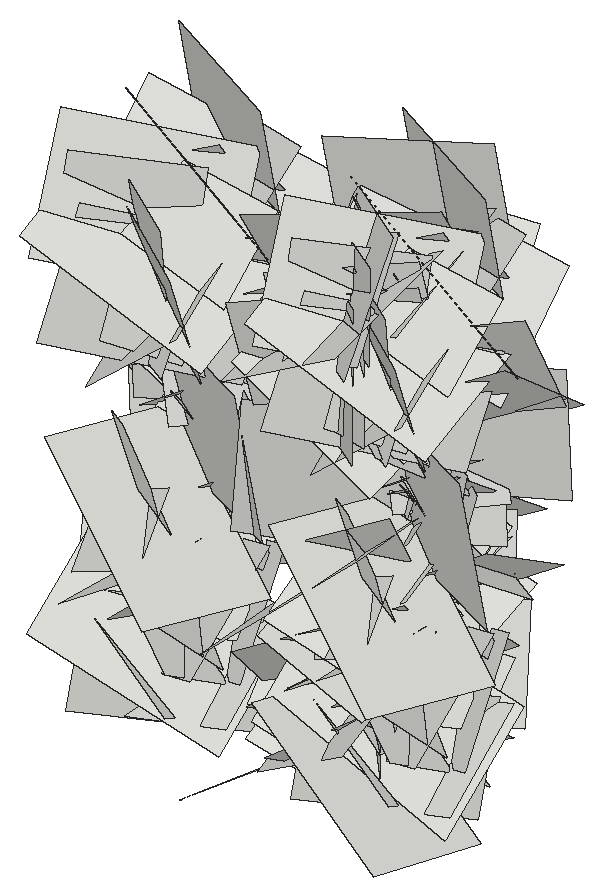
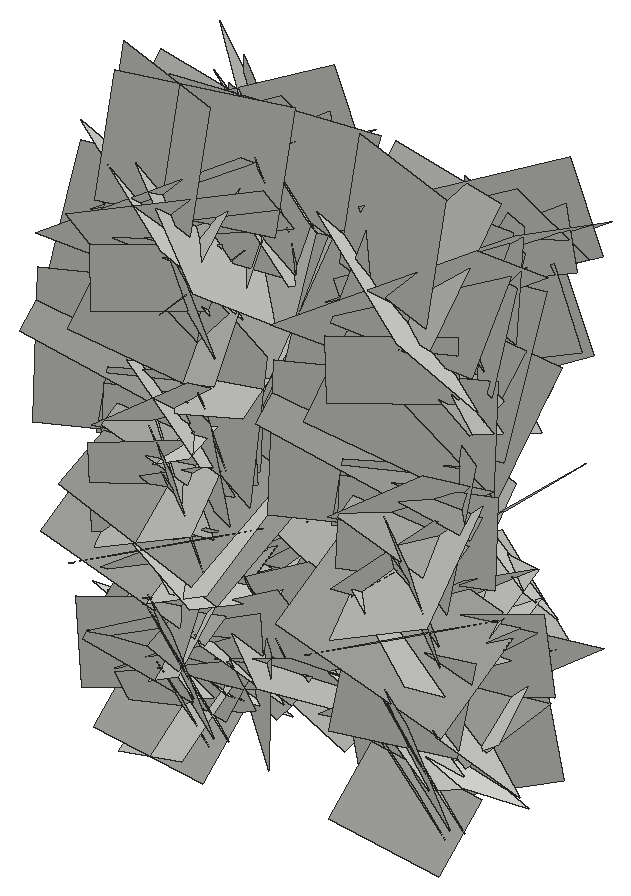
# SketchUp Ruby script. Lengths in inches.
U = 1.inch
M = Sketchup.active_model
def pt(a) = Geom::Point3d.new(a.map { |v| v * U })
def face(e, loops, mat)
  f = e.add_face(loops[0].map { |a| pt(a) })
  loops[1..].each { |l| e.add_face(l.map { |a| pt(a) }).erase! }
  f.material = f.back_material = mat if mat
  f
end
# faces: each face lists its corners as indices into pts; further lists are holes
def faces(e, pts, list, mat = nil) = list.each { |f| face(e, (f[0].is_a?(Array) ? f : [f]).map { |l| l.map { |i| pts[i] } }, mat) }
# xy, xz, yz: faces in a plane at the given z, y or x. An outline is a flat list of corners, or four numbers for a rectangle; further outlines are holes
def ring(l) = l.size == 4 ? [[l[0], l[1]], [l[2], l[1]], [l[2], l[3]], [l[0], l[3]]] : l.each_slice(2).to_a
def flat(e, list, mat, &to3) = list.each { |f| face(e, (f[0].is_a?(Array) ? f : [f]).map { |l| ring(l).map { |u, v| to3.(u, v) } }, mat) }
def xy(e, z, list, mat = nil) = flat(e, list, mat) { |x, y| [x, y, z] }
def xz(e, y, list, mat = nil) = flat(e, list, mat) { |x, z| [x, y, z] }
def yz(e, x, list, mat = nil) = flat(e, list, mat) { |y, z| [x, y, z] }
def lines(e, pts, list) = list.each { |a, b| e.add_line(pt(pts[a]), pt(pts[b])) }
# prism: a flat outline (further loops are holes) pulled along v
def prism(e, loops, v, mat = nil)
  f = face(e, loops, mat); d = Geom::Vector3d.new(v.map { |x| x * U })
  f.pushpull(f.normal.samedirection?(d) ? d.length : -d.length)
end
def box(e, o, s, mat = nil) = prism(e, [[o, [o[0] + s[0], o[1], o[2]], [o[0] + s[0], o[1] + s[1], o[2]], [o[0], o[1] + s[1], o[2]]]], [0, 0, s[2]], mat)
def at(x, y, z, deg = 0) = Geom::Transformation.translation(pt([x, y, z])) * Geom::Transformation.rotation(ORIGIN, Z_AXIS, deg.degrees)
def axes(o, x, y, z) = Geom::Transformation.new([*x, 0, *y, 0, *z, 0, *pt(o).to_a, 1])
def part(name) = M.definitions.add(name)
# library, detail: a bought-in or finely detailed component or shape, given as its bounding box
def library(name, o, s) = part(name).tap { |d| box(d.entities, o, s) }
def detail(e, o, s) = box(e.add_group.entities, o, s)
def put(e, d, t, mat = nil) = e.add_instance(d, t).tap { |i| i.material = mat if mat }
def group(e, t, mat = nil) = e.add_group.tap { |g| g.transformation = t; g.material = mat if mat }.entities
root = M.entities
c1 = part("Component\#6")
p = [[0.01,0,0],[0,3.24,4.54],[4.32,3.24,4.54],[4.33,0,0]]
faces(c1.entities,p,[[0,1,2,3]])
put(root,c1,axes([424.49,200.25,4.79],[-0.06637,1.27776,-0.24675],[0.01199,-0.2465,-1.2793],[-1.3794,-0.06362,0.00075]))
put(root,c1,axes([420.52,200.25,4.79],[0.06637,1.27776,-0.24675],[-0.01199,-0.2465,-1.2793],[1.3794,-0.06362,0.00075]))
put(root,c1,axes([410.71,204.41,7.91],[0.10208,-0.52254,-0.48763],[0.08086,-0.48171,0.53127],[0.75328,0.12252,0.00905]))
put(root,c1,axes([424.49,204.41,7.91],[-0.10208,-0.52254,-0.48763],[-0.08086,-0.48171,0.53127],[-0.75328,0.12252,0.00905]))
put(root,c1,axes([420.52,204.41,7.91],[0.10208,-0.52254,-0.48763],[0.08086,-0.48171,0.53127],[0.75328,0.12252,0.00905]))
put(root,c1,axes([414.68,200.61,7.25],[0.15258,0.77944,0.1154],[0.02035,0.1138,-0.79262],[-0.83497,0.14521,0.00177]))
put(root,c1,axes([420.52,200.61,7.25],[-0.15258,0.77944,0.1154],[-0.02035,0.1138,-0.79262],[0.83497,0.14521,0.00177]))
put(root,c1,axes([424.49,200.61,7.25],[0.15258,0.77944,0.1154],[0.02035,0.1138,-0.79262],[-0.83497,0.14521,0.00177]))
put(root,c1,axes([410.71,201.43,15.61],[0.13511,0.17275,0.7909],[0.07376,0.79534,-0.18493],[0.85494,-0.09592,-0.10904]))
put(root,c1,axes([424.49,201.43,15.61],[-0.13511,0.17275,0.7909],[-0.07376,0.79534,-0.18493],[-0.85494,-0.09592,-0.10904]))
put(root,c1,axes([420.52,201.43,15.61],[0.13511,0.17275,0.7909],[0.07376,0.79534,-0.18493],[0.85494,-0.09592,-0.10904]))
put(root,c1,axes([410.71,201.2,11.35],[0.2643,1.29708,-0.17492],[-0.19217,-0.14212,-1.31229],[1.37397,-0.26938,-0.1499]))
put(root,c1,axes([424.49,201.2,11.35],[-0.2643,1.29708,-0.17492],[0.19217,-0.14212,-1.31229],[-1.37397,-0.26938,-0.1499]))
put(root,c1,axes([420.52,201.2,11.35],[0.2643,1.29708,-0.17492],[-0.19217,-0.14212,-1.31229],[1.37397,-0.26938,-0.1499]))
put(root,c1,axes([410.71,201.6875,18.6875],[0.06388,0.10125,0.82658],[-0.05301,0.82768,-0.09774],[0.88113,0.04245,-0.0658]))
put(root,c1,axes([424.49,201.6875,18.6875],[-0.06388,0.10125,0.82658],[0.05301,0.82768,-0.09774],[-0.88113,0.04245,-0.0658]))
put(root,c1,axes([420.52,201.6875,18.6875],[0.06388,0.10125,0.82658],[-0.05301,0.82768,-0.09774],[0.88113,0.04245,-0.0658]))
put(root,c1,axes([410.71,204.39,20.61],[0.01972,0.37325,-1.09096],[0.03348,-1.09086,-0.37268],[1.22177,0.02387,0.02782]))
put(root,c1,axes([424.49,204.39,20.61],[-0.01972,0.37325,-1.09096],[-0.03348,-1.09086,-0.37268],[-1.22177,0.02387,0.02782]))
put(root,c1,axes([420.52,204.39,20.61],[0.01972,0.37325,-1.09096],[0.03348,-1.09086,-0.37268],[1.22177,0.02387,0.02782]))
put(root,c1,axes([410.71,199.86,19.8],[-0.08167,1.25653,0.46028],[0.00634,0.46136,-1.25848],[1.41846,0.07029,0.03212]))
put(root,c1,axes([424.49,199.86,19.8],[0.08167,1.25653,0.46028],[-0.00634,0.46136,-1.25848],[-1.41846,0.07029,0.03212]))
put(root,c1,axes([420.52,199.86,19.8],[-0.08167,1.25653,0.46028],[0.00634,0.46136,-1.25848],[1.41846,0.07029,0.03212]))
put(root,c1,axes([414.68,203.18,8],[-0.06036,-0.35202,0.5516],[0.07606,0.54699,0.35648],[-0.68943,0.09116,-0.00896]))
put(root,c1,axes([420.52,203.18,8],[0.06036,-0.35202,0.5516],[-0.07606,0.54699,0.35648],[0.68943,0.09116,-0.00896]))
put(root,c1,axes([424.49,203.18,8],[-0.06036,-0.35202,0.5516],[0.07606,0.54699,0.35648],[-0.68943,0.09116,-0.00896]))
put(root,c1,axes([410.71,204.45,21.63],[-0.07523,0.18922,-0.91056],[0.04715,-0.91147,-0.19287],[0.98469,0.0581,-0.06033]))
put(root,c1,axes([424.49,204.45,21.63],[0.07523,0.18922,-0.91056],[-0.04715,-0.91147,-0.19287],[-0.98469,0.0581,-0.06033]))
put(root,c1,axes([420.52,204.45,21.63],[-0.07523,0.18922,-0.91056],[0.04715,-0.91147,-0.19287],[0.98469,0.0581,-0.06033]))
put(root,c1,axes([410.71,203.64,8.5],[0.20575,0.76434,-0.74551],[-0.06488,-0.74852,-0.78336],[1.12991,-0.18216,0.09078]))
put(root,c1,axes([424.49,203.64,8.5],[-0.20575,0.76434,-0.74551],[0.06488,-0.74852,-0.78336],[-1.12991,-0.18216,0.09078]))
put(root,c1,axes([420.52,203.64,8.5],[0.20575,0.76434,-0.74551],[-0.06488,-0.74852,-0.78336],[1.12991,-0.18216,0.09078]))
put(root,c1,axes([410.71,201.07,18.92],[0.13602,0.69446,0.8684],[0.06726,0.86816,-0.70365],[1.17673,-0.1299,-0.06016]))
put(root,c1,axes([424.49,201.07,18.92],[-0.13602,0.69446,0.8684],[-0.06726,0.86816,-0.70365],[-1.17673,-0.1299,-0.06016]))
put(root,c1,axes([420.52,201.07,18.92],[0.13602,0.69446,0.8684],[0.06726,0.86816,-0.70365],[1.17673,-0.1299,-0.06016]))
put(root,c1,axes([410.71,200.34,18.7],[-0.08817,0.51183,1.11442],[-0.20058,1.09825,-0.51853],[1.28435,0.20665,-0.00447]))
put(root,c1,axes([424.49,200.34,18.7],[0.08817,0.51183,1.11442],[0.20058,1.09825,-0.51853],[-1.28435,0.20665,-0.00447]))
put(root,c1,axes([420.52,200.34,18.7],[-0.08817,0.51183,1.11442],[-0.20058,1.09825,-0.51853],[1.28435,0.20665,-0.00447]))
put(root,c1,axes([410.71,200.79,15.19],[0.21334,0.28139,1.2169],[-0.22593,1.22225,-0.24738],[1.30453,0.16566,-0.24185]))
put(root,c1,axes([424.49,200.79,15.19],[-0.21334,0.28139,1.2169],[0.22593,1.22225,-0.24738],[-1.30453,0.16566,-0.24185]))
put(root,c1,axes([420.52,200.79,15.19],[0.21334,0.28139,1.2169],[-0.22593,1.22225,-0.24738],[1.30453,0.16566,-0.24185]))
put(root,c1,axes([414.68,205.06,0.06],[0.16762,-0.72435,0.3647],[0.00744,0.37278,0.73735],[-0.85961,-0.13802,0.0775]))
put(root,c1,axes([420.52,205.06,0.06],[-0.16762,-0.72435,0.3647],[-0.00744,0.37278,0.73735],[0.85961,-0.13802,0.0775]))
put(root,c1,axes([424.49,205.06,0.06],[0.16762,-0.72435,0.3647],[0.00744,0.37278,0.73735],[-0.85961,-0.13802,0.0775]))
put(root,c1,axes([414.68,202.62,14.39],[0.09007,0.1944,0.61889],[-0.03503,0.62466,-0.19168],[-0.68673,-0.00637,0.09095]))
put(root,c1,axes([420.52,202.62,14.39],[-0.09007,0.1944,0.61889],[0.03503,0.62466,-0.19168],[0.68673,-0.00637,0.09095]))
put(root,c1,axes([424.49,202.62,14.39],[0.09007,0.1944,0.61889],[-0.03503,0.62466,-0.19168],[-0.68673,-0.00637,0.09095]))
put(root,c1,axes([410.71,200.25,4.04],[-0.10038,1.14624,0.70824],[-0.13093,0.69961,-1.1488],[1.42222,0.14531,-0.05578]))
put(root,c1,axes([424.49,200.25,4.04],[0.10038,1.14624,0.70824],[0.13093,0.69961,-1.1488],[-1.42222,0.14531,-0.05578]))
put(root,c1,axes([420.52,200.25,4.04],[-0.10038,1.14624,0.70824],[-0.13093,0.69961,-1.1488],[1.42222,0.14531,-0.05578]))
put(root,c1,axes([410.71,207.09,15.04],[0.15807,-1.02909,-0.4958],[-0.14338,-0.5124,1.02286],[1.20232,0.07419,0.18716]))
put(root,c1,axes([424.49,207.09,15.04],[-0.15807,-1.02909,-0.4958],[0.14338,-0.5124,1.02286],[-1.20232,0.07419,0.18716]))
put(root,c1,axes([420.52,207.09,15.04],[0.15807,-1.02909,-0.4958],[-0.14338,-0.5124,1.02286],[1.20232,0.07419,0.18716]))
put(root,c1,axes([414.68,205.68,16.84],[-0.07036,-0.63328,-0.02287],[0.09357,-0.03201,0.6302],[-0.66517,0.06248,0.09107]))
put(root,c1,axes([420.52,205.68,16.84],[0.07036,-0.63328,-0.02287],[-0.09357,-0.03201,0.6302],[0.66517,0.06248,0.09107]))
put(root,c1,axes([424.49,205.68,16.84],[-0.07036,-0.63328,-0.02287],[0.09357,-0.03201,0.6302],[-0.66517,0.06248,0.09107]))
put(root,c1,axes([414.68,203.04,6.2],[0.19197,0.78573,-0.28472],[0.09491,-0.3079,-0.79273],[-0.88077,0.13807,-0.14748]))
put(root,c1,axes([420.52,203.04,6.2],[-0.19197,0.78573,-0.28472],[-0.09491,-0.3079,-0.79273],[0.88077,0.13807,-0.14748]))
put(root,c1,axes([424.49,203.04,6.2],[0.19197,0.78573,-0.28472],[0.09491,-0.3079,-0.79273],[-0.88077,0.13807,-0.14748]))
put(root,c1,axes([410.71,203.52,7.375],[0.0121,1.00291,-0.55649],[-0.12117,-0.55275,-0.99852],[1.20972,-0.0654,-0.09445]))
put(root,c1,axes([424.49,203.52,7.375],[-0.0121,1.00291,-0.55649],[0.12117,-0.55275,-0.99852],[-1.20972,-0.0654,-0.09445]))
put(root,c1,axes([420.52,203.52,7.375],[0.0121,1.00291,-0.55649],[-0.12117,-0.55275,-0.99852],[1.20972,-0.0654,-0.09445]))
put(root,c1,axes([410.71,202.39,0.06],[0.12593,0.12266,1.10922],[-0.15067,1.10807,-0.10731],[1.17331,0.12913,-0.13284]))
put(root,c1,axes([424.49,202.39,0.06],[-0.12593,0.12266,1.10922],[0.15067,1.10807,-0.10731],[-1.17331,0.12913,-0.13284]))
put(root,c1,axes([420.52,202.39,0.06],[0.12593,0.12266,1.10922],[-0.15067,1.10807,-0.10731],[1.17331,0.12913,-0.13284]))
put(root,c1,axes([410.71,202.81,3.34],[-0.17899,0.36268,0.93898],[0.06935,0.95405,-0.35673],[1.06473,-0.00117,0.18108]))
put(root,c1,axes([424.49,202.81,3.34],[0.17899,0.36268,0.93898],[-0.06935,0.95405,-0.35673],[-1.06473,-0.00117,0.18108]))
put(root,c1,axes([420.52,202.81,3.34],[-0.17899,0.36268,0.93898],[0.06935,0.95405,-0.35673],[1.06473,-0.00117,0.18108]))
put(root,c1,axes([410.71,203.75,8.58],[0.14047,0.70659,0.15459],[-0.00867,0.15861,-0.71798],[0.76665,-0.12767,-0.03644]))
put(root,c1,axes([424.49,203.75,8.58],[-0.14047,0.70659,0.15459],[0.00867,0.15861,-0.71798],[-0.76665,-0.12767,-0.03644]))
put(root,c1,axes([420.52,203.75,8.58],[0.14047,0.70659,0.15459],[-0.00867,0.15861,-0.71798],[0.76665,-0.12767,-0.03644]))
put(root,c1,axes([410.71,206.9375,13.83],[0.19711,0.10382,-1.30915],[0.13395,-1.31749,-0.08653],[1.38559,0.11259,0.1946]))
put(root,c1,axes([424.49,206.9375,13.83],[-0.19711,0.10382,-1.30915],[-0.13395,-1.31749,-0.08653],[-1.38559,0.11259,0.1946]))
put(root,c1,axes([420.52,206.9375,13.83],[0.19711,0.10382,-1.30915],[0.13395,-1.31749,-0.08653],[1.38559,0.11259,0.1946]))
put(root,c1,axes([410.71,207.71,2.15],[0.07423,-0.90085,-0.6111],[0.34403,-0.56723,0.87337],[1.1014,0.23789,-0.23162]))
put(root,c1,axes([424.49,207.71,2.15],[-0.07423,-0.90085,-0.6111],[-0.34403,-0.56723,0.87337],[-1.1014,0.23789,-0.23162]))
put(root,c1,axes([420.52,207.71,2.15],[0.07423,-0.90085,-0.6111],[0.34403,-0.56723,0.87337],[1.1014,0.23789,-0.23162]))
put(root,c1,axes([414.68,204.05,18.57],[-0.06151,0.80519,-0.14469],[0.18353,-0.12968,-0.7911],[-0.84753,-0.08652,-0.16081]))
put(root,c1,axes([420.52,204.05,18.57],[0.06151,0.80519,-0.14469],[-0.18353,-0.12968,-0.7911],[0.84753,-0.08652,-0.16081]))
put(root,c1,axes([424.49,204.05,18.57],[-0.06151,0.80519,-0.14469],[0.18353,-0.12968,-0.7911],[-0.84753,-0.08652,-0.16081]))
put(root,c1,axes([410.71,209.01,4.56],[-0.09462,-0.88739,-0.86898],[0.02241,-0.87218,0.88849],[1.31634,-0.04894,-0.07759]))
put(root,c1,axes([424.49,209.01,4.56],[0.09462,-0.88739,-0.86898],[-0.02241,-0.87218,0.88849],[-1.31634,-0.04894,-0.07759]))
put(root,c1,axes([420.52,209.01,4.56],[-0.09462,-0.88739,-0.86898],[0.02241,-0.87218,0.88849],[1.31634,-0.04894,-0.07759]))
put(root,c1,axes([414.68,205.78,22.17],[-0.00372,0.37911,-0.54343],[-0.01311,-0.54338,-0.37899],[-0.70223,0.00813,0.00995]))
put(root,c1,axes([420.52,205.78,22.17],[0.00372,0.37911,-0.54343],[0.01311,-0.54338,-0.37899],[0.70223,0.00813,0.00995]))
put(root,c1,axes([424.49,205.78,22.17],[-0.00372,0.37911,-0.54343],[-0.01311,-0.54338,-0.37899],[-0.70223,0.00813,0.00995]))
put(root,c1,axes([410.71,205.65,23.04],[0.12198,0.70336,-1.01008],[0.22842,-1.01033,-0.67899],[1.28455,0.11286,0.21665]))
put(root,c1,axes([424.49,205.65,23.04],[-0.12198,0.70336,-1.01008],[-0.22842,-1.01033,-0.67899],[-1.28455,0.11286,0.21665]))
put(root,c1,axes([420.52,205.65,23.04],[0.12198,0.70336,-1.01008],[0.22842,-1.01033,-0.67899],[1.28455,0.11286,0.21665]))
put(root,c1,axes([410.71,205.49,13.28],[0.13832,-0.68419,1.12815],[0.08396,1.13567,0.67959],[1.39605,-0.00051,-0.15265]))
put(root,c1,axes([424.49,205.49,13.28],[-0.13832,-0.68419,1.12815],[-0.08396,1.13567,0.67959],[-1.39605,-0.00051,-0.15265]))
put(root,c1,axes([420.52,205.49,13.28],[0.13832,-0.68419,1.12815],[0.08396,1.13567,0.67959],[1.39605,-0.00051,-0.15265]))
put(root,c1,axes([410.71,206.11,11.76],[-0.09648,-0.72051,0.9522],[-0.19874,0.95174,0.70224],[1.25002,0.0957,0.18514]))
put(root,c1,axes([424.49,206.11,11.76],[0.09648,-0.72051,0.9522],[0.19874,0.95174,0.70224],[-1.25002,0.0957,0.18514]))
put(root,c1,axes([420.52,206.11,11.76],[-0.09648,-0.72051,0.9522],[-0.19874,0.95174,0.70224],[1.25002,0.0957,0.18514]))
put(root,c1,axes([410.71,207.28,11.15],[0.07738,-1.09853,0.81062],[0.01823,0.81245,1.09947],[1.44703,0.04851,-0.0572]))
put(root,c1,axes([424.49,207.28,11.15],[-0.07738,-1.09853,0.81062],[-0.01823,0.81245,1.09947],[-1.44703,0.04851,-0.0572]))
put(root,c1,axes([420.52,207.28,11.15],[0.07738,-1.09853,0.81062],[0.01823,0.81245,1.09947],[1.44703,0.04851,-0.0572]))
put(root,c1,axes([410.71,207.17,17.14],[0.0563,-0.55845,0.63654],[0.00808,0.63808,0.55916],[0.89756,0.02928,-0.04497]))
put(root,c1,axes([424.49,207.17,17.14],[-0.0563,-0.55845,0.63654],[-0.00808,0.63808,0.55916],[-0.89756,0.02928,-0.04497]))
put(root,c1,axes([420.52,207.17,17.14],[0.0563,-0.55845,0.63654],[0.00808,0.63808,0.55916],[0.89756,0.02928,-0.04497]))
put(root,c1,axes([410.71,203.17,19.17],[-0.16233,1.06667,0.75788],[-0.09967,0.75211,-1.07754],[1.38342,0.17935,0.0113]))
put(root,c1,axes([424.49,203.17,19.17],[0.16233,1.06667,0.75788],[0.09967,0.75211,-1.07754],[-1.38342,0.17935,0.0113]))
put(root,c1,axes([420.52,203.17,19.17],[-0.16233,1.06667,0.75788],[-0.09967,0.75211,-1.07754],[1.38342,0.17935,0.0113]))
put(root,c1,axes([410.71,209.96,4.13],[0.07876,-0.66244,-0.94852],[0.03994,-0.94858,0.66543],[1.2257,0.07348,0.03927]))
put(root,c1,axes([424.49,209.96,4.13],[-0.07876,-0.66244,-0.94852],[-0.03994,-0.94858,0.66543],[-1.2257,0.07348,0.03927]))
put(root,c1,axes([420.52,209.96,4.13],[0.07876,-0.66244,-0.94852],[0.03994,-0.94858,0.66543],[1.2257,0.07348,0.03927]))
put(root,c1,axes([414.68,209.54,8.98],[-0.01886,-0.65319,-0.4186],[0.2021,-0.40955,0.63097],[-0.79714,-0.08839,0.16987]))
put(root,c1,axes([420.52,209.54,8.98],[0.01886,-0.65319,-0.4186],[-0.2021,-0.40955,0.63097],[0.79714,-0.08839,0.16987]))
put(root,c1,axes([424.49,209.54,8.98],[-0.01886,-0.65319,-0.4186],[0.2021,-0.40955,0.63097],[-0.79714,-0.08839,0.16987]))
put(root,c1,axes([414.68,205.65,3.3125],[-0.06993,0.62057,0.27964],[-0.0119,0.27992,-0.62384],[-0.72141,-0.06477,-0.01682]))
put(root,c1,axes([420.52,205.65,3.3125],[0.06993,0.62057,0.27964],[0.0119,0.27992,-0.62384],[0.72141,-0.06477,-0.01682]))
put(root,c1,axes([424.49,205.65,3.3125],[-0.06993,0.62057,0.27964],[-0.0119,0.27992,-0.62384],[-0.72141,-0.06477,-0.01682]))
put(root,c1,axes([414.68,208.89,13.53],[0.18208,-0.09561,-0.67164],[0.05748,-0.68868,0.1119],[-0.71681,-0.07951,-0.16163]))
put(root,c1,axes([420.52,208.89,13.53],[-0.18208,-0.09561,-0.67164],[-0.05748,-0.68868,0.1119],[0.71681,-0.07951,-0.16163]))
put(root,c1,axes([424.49,208.89,13.53],[0.18208,-0.09561,-0.67164],[0.05748,-0.68868,0.1119],[-0.71681,-0.07951,-0.16163]))
put(root,c1,axes([410.71,205.98,8.7],[-0.1184,0.10295,0.88925],[0.12891,0.88959,-0.08771],[0.94011,-0.10902,0.12403]))
put(root,c1,axes([424.49,205.98,8.7],[0.1184,0.10295,0.88925],[-0.12891,0.88959,-0.08771],[-0.94011,-0.10902,0.12403]))
put(root,c1,axes([420.52,205.98,8.7],[-0.1184,0.10295,0.88925],[0.12891,0.88959,-0.08771],[0.94011,-0.10902,0.12403]))
put(root,c1,axes([420.52,207.72,1.15],[-0.00392,-0.70388,0.63123],[-0.16138,0.62344,0.69431],[0.98911,0.09893,0.11578]))
put(root,c1,axes([424.49,207.72,1.15],[0.00392,-0.70388,0.63123],[0.16138,0.62344,0.69431],[-0.98911,0.09893,0.11578]))
put(root,c1,axes([410.71,208.78,4.43],[0.01106,-0.99025,0.53374],[0.00744,0.53381,0.99025],[1.19241,0.00586,-0.01113]))
put(root,c1,axes([424.49,208.78,4.43],[-0.01106,-0.99025,0.53374],[-0.00744,0.53381,0.99025],[-1.19241,0.00586,-0.01113]))
put(root,c1,axes([420.52,208.78,4.43],[0.01106,-0.99025,0.53374],[0.00744,0.53381,0.99025],[1.19241,0.00586,-0.01113]))
put(root,c1,axes([414.68,206.67,12.85],[-0.04142,0.63331,-0.27554],[-0.00251,-0.27611,-0.63426],[-0.73209,-0.03488,0.01776]))
put(root,c1,axes([420.52,206.67,12.85],[0.04142,0.63331,-0.27554],[0.00251,-0.27611,-0.63426],[0.73209,-0.03488,0.01776]))
put(root,c1,axes([424.49,206.67,12.85],[-0.04142,0.63331,-0.27554],[-0.00251,-0.27611,-0.63426],[-0.73209,-0.03488,0.01776]))
put(root,c1,axes([410.71,206.09,10.75],[0.05447,-0.13377,1.26127],[0.13355,1.2566,0.12815],[1.33779,-0.12,-0.06414]))
put(root,c1,axes([424.49,206.09,10.75],[-0.05447,-0.13377,1.26127],[-0.13355,1.2566,0.12815],[-1.33779,-0.12,-0.06414]))
put(root,c1,axes([420.52,206.09,10.75],[0.05447,-0.13377,1.26127],[0.13355,1.2566,0.12815],[1.33779,-0.12,-0.06414]))
put(root,c1,axes([410.71,206,12.43],[0.16769,0.64159,0.3622],[-0.01184,0.3725,-0.65496],[0.78088,-0.13213,-0.08771]))
put(root,c1,axes([424.49,206,12.43],[-0.16769,0.64159,0.3622],[0.01184,0.3725,-0.65496],[-0.78088,-0.13213,-0.08771]))
put(root,c1,axes([420.52,206,12.43],[0.16769,0.64159,0.3622],[-0.01184,0.3725,-0.65496],[0.78088,-0.13213,-0.08771]))
put(root,c1,axes([414.68,206.15,0.87],[0.01906,0.33732,0.58365],[-0.0637,0.58234,-0.33471],[-0.71172,-0.04309,0.04558]))
put(root,c1,axes([420.52,206.15,0.87],[-0.01906,0.33732,0.58365],[0.0637,0.58234,-0.33471],[0.71172,-0.04309,0.04558]))
put(root,c1,axes([424.49,206.15,0.87],[0.01906,0.33732,0.58365],[-0.0637,0.58234,-0.33471],[-0.71172,-0.04309,0.04558]))
put(root,c1,axes([410.71,208.53,24.44],[0.00063,0.23668,-1.01361],[0.18606,-0.99912,-0.23319],[1.08753,0.17079,0.04049]))
put(root,c1,axes([424.49,208.53,24.44],[-0.00063,0.23668,-1.01361],[-0.18606,-0.99912,-0.23319],[-1.08753,0.17079,0.04049]))
put(root,c1,axes([420.52,208.53,24.44],[0.00063,0.23668,-1.01361],[0.18606,-0.99912,-0.23319],[1.08753,0.17079,0.04049]))
put(root,c1,axes([414.68,206.6,8.35],[-0.07615,0.29672,0.54367],[-0.07213,0.54022,-0.30383],[-0.65256,-0.09434,-0.02986]))
put(root,c1,axes([424.49,206.6,8.35],[-0.07615,0.29672,0.54367],[-0.07213,0.54022,-0.30383],[-0.65256,-0.09434,-0.02986]))
put(root,c1,axes([420.52,206.6,8.35],[0.07615,0.29672,0.54367],[0.07213,0.54022,-0.30383],[0.65256,-0.09434,-0.02986]))
put(root,c1,axes([410.71,211.08,20.1875],[-0.1855,-0.74932,-0.85781],[0.09412,-0.87421,0.74553],[1.20366,-0.04712,-0.19049]))
put(root,c1,axes([424.49,211.08,20.1875],[0.1855,-0.74932,-0.85781],[-0.09412,-0.87421,0.74553],[-1.20366,-0.04712,-0.19049]))
put(root,c1,axes([420.52,211.08,20.1875],[-0.1855,-0.74932,-0.85781],[0.09412,-0.87421,0.74553],[1.20366,-0.04712,-0.19049]))
put(root,c1,axes([410.71,206.49,12.28],[-0.17995,0.92169,-0.62911],[0.1265,-0.6177,-0.93718],[1.17609,0.20746,0.00455]))
put(root,c1,axes([424.49,206.49,12.28],[0.17995,0.92169,-0.62911],[-0.1265,-0.6177,-0.93718],[-1.17609,0.20746,0.00455]))
put(root,c1,axes([420.52,206.49,12.28],[-0.17995,0.92169,-0.62911],[0.1265,-0.6177,-0.93718],[1.17609,0.20746,0.00455]))
put(root,c1,axes([414.68,206.02,7.14],[-0.00935,0.6115,0.38278],[0.02819,0.38283,-0.61096],[-0.76419,0.00664,-0.02722]))
put(root,c1,axes([420.52,206.02,7.14],[0.00935,0.6115,0.38278],[-0.02819,0.38283,-0.61096],[0.76419,0.00664,-0.02722]))
put(root,c1,axes([424.49,206.02,7.14],[-0.00935,0.6115,0.38278],[0.02819,0.38283,-0.61096],[-0.76419,0.00664,-0.02722]))
put(root,c1,axes([414.68,207.38,2.3],[-0.03327,0.56132,-0.40527],[-0.08729,-0.40584,-0.55572],[-0.72866,0.02299,0.08508]))
put(root,c1,axes([420.52,207.38,2.3],[0.03327,0.56132,-0.40527],[0.08729,-0.40584,-0.55572],[0.72866,0.02299,0.08508]))
put(root,c1,axes([424.49,207.38,2.3],[-0.03327,0.56132,-0.40527],[-0.08729,-0.40584,-0.55572],[-0.72866,0.02299,0.08508]))
put(root,c1,axes([410.71,205.78,7.5],[-0.02909,0.83454,0.28231],[0.13137,0.2833,-0.8254],[0.92457,-0.01399,0.12617]))
put(root,c1,axes([424.49,205.78,7.5],[0.02909,0.83454,0.28231],[-0.13137,0.2833,-0.8254],[-0.92457,-0.01399,0.12617]))
put(root,c1,axes([420.52,205.78,7.5],[-0.02909,0.83454,0.28231],[0.13137,0.2833,-0.8254],[0.92457,-0.01399,0.12617]))
put(root,c1,axes([414.68,205.95,7.64],[0.13368,0.21915,0.90835],[0.05222,0.91375,-0.2273],[-0.9891,0.07786,0.11076]))
put(root,c1,axes([420.52,205.95,7.64],[-0.13368,0.21915,0.90835],[-0.05222,0.91375,-0.2273],[0.9891,0.07786,0.11076]))
put(root,c1,axes([424.49,205.95,7.64],[0.13368,0.21915,0.90835],[0.05222,0.91375,-0.2273],[-0.9891,0.07786,0.11076]))
put(root,c1,axes([414.68,209.83,18.53],[0.13516,-0.18826,-0.70807],[0.00477,-0.7185,0.19184],[-0.77662,-0.03718,-0.12206]))
put(root,c1,axes([420.52,209.83,18.53],[-0.13516,-0.18826,-0.70807],[-0.00477,-0.7185,0.19184],[0.77662,-0.03718,-0.12206]))
put(root,c1,axes([424.49,209.83,18.53],[0.13516,-0.18826,-0.70807],[0.00477,-0.7185,0.19184],[-0.77662,-0.03718,-0.12206]))
put(root,c1,axes([410.71,210.56,5.71],[-0.17873,-0.295,-0.9769],[0.02803,-0.99107,0.29472],[1.08133,-0.02307,-0.16911]))
put(root,c1,axes([424.49,210.56,5.71],[0.17873,-0.295,-0.9769],[-0.02803,-0.99107,0.29472],[-1.08133,-0.02307,-0.16911]))
put(root,c1,axes([420.52,210.56,5.71],[-0.17873,-0.295,-0.9769],[0.02803,-0.99107,0.29472],[1.08133,-0.02307,-0.16911]))
put(root,c1,axes([414.68,208.64,6.82],[-0.0498,0.28937,-0.67344],[-0.06797,-0.67386,-0.28508],[-0.77398,0.04056,0.06836]))
put(root,c1,axes([420.52,208.64,6.82],[0.0498,0.28937,-0.67344],[0.06797,-0.67386,-0.28508],[0.77398,0.04056,0.06836]))
